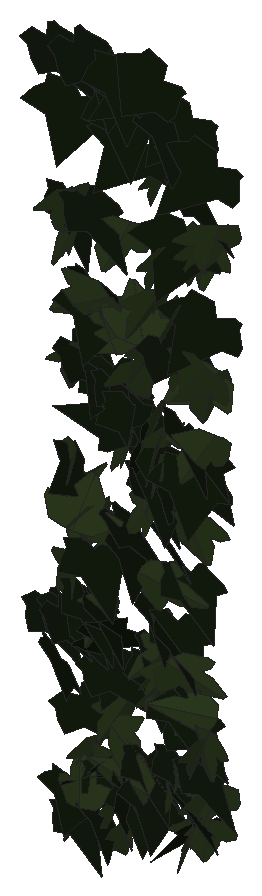
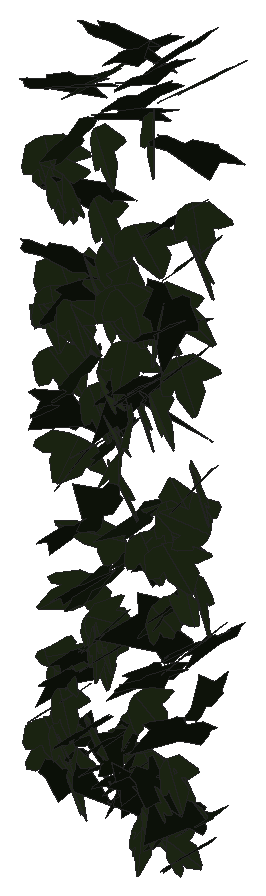
# SketchUp Ruby script. Lengths in inches.
U = 1.inch
M = Sketchup.active_model
def pt(a) = Geom::Point3d.new(a.map { |v| v * U })
def face(e, loops, mat)
  f = e.add_face(loops[0].map { |a| pt(a) })
  loops[1..].each { |l| e.add_face(l.map { |a| pt(a) }).erase! }
  f.material = f.back_material = mat if mat
  f
end
# faces: each face lists its corners as indices into pts; further lists are holes
def faces(e, pts, list, mat = nil) = list.each { |f| face(e, (f[0].is_a?(Array) ? f : [f]).map { |l| l.map { |i| pts[i] } }, mat) }
# xy, xz, yz: faces in a plane at the given z, y or x. An outline is a flat list of corners, or four numbers for a rectangle; further outlines are holes
def ring(l) = l.size == 4 ? [[l[0], l[1]], [l[2], l[1]], [l[2], l[3]], [l[0], l[3]]] : l.each_slice(2).to_a
def flat(e, list, mat, &to3) = list.each { |f| face(e, (f[0].is_a?(Array) ? f : [f]).map { |l| ring(l).map { |u, v| to3.(u, v) } }, mat) }
def xy(e, z, list, mat = nil) = flat(e, list, mat) { |x, y| [x, y, z] }
def xz(e, y, list, mat = nil) = flat(e, list, mat) { |x, z| [x, y, z] }
def yz(e, x, list, mat = nil) = flat(e, list, mat) { |y, z| [x, y, z] }
def lines(e, pts, list) = list.each { |a, b| e.add_line(pt(pts[a]), pt(pts[b])) }
# prism: a flat outline (further loops are holes) pulled along v
def prism(e, loops, v, mat = nil)
  f = face(e, loops, mat); d = Geom::Vector3d.new(v.map { |x| x * U })
  f.pushpull(f.normal.samedirection?(d) ? d.length : -d.length)
end
def box(e, o, s, mat = nil) = prism(e, [[o, [o[0] + s[0], o[1], o[2]], [o[0] + s[0], o[1] + s[1], o[2]], [o[0], o[1] + s[1], o[2]]]], [0, 0, s[2]], mat)
def at(x, y, z, deg = 0) = Geom::Transformation.translation(pt([x, y, z])) * Geom::Transformation.rotation(ORIGIN, Z_AXIS, deg.degrees)
def axes(o, x, y, z) = Geom::Transformation.new([*x, 0, *y, 0, *z, 0, *pt(o).to_a, 1])
def part(name) = M.definitions.add(name)
# library, detail: a bought-in or finely detailed component or shape, given as its bounding box
def library(name, o, s) = part(name).tap { |d| box(d.entities, o, s) }
def detail(e, o, s) = box(e.add_group.entities, o, s)
def put(e, d, t, mat = nil) = e.add_instance(d, t).tap { |i| i.material = mat if mat }
def group(e, t, mat = nil) = e.add_group.tap { |g| g.transformation = t; g.material = mat if mat }.entities
root = M.entities
M.materials.add("1026 AP 7946 SUNNY SIDE UP").color = [254, 231, 186]
M.materials.add("efeu1").color = [18, 25, 13]
M.materials.add("efeu2").color = [43, 57, 29]
c1 = part("ivyleaf_9")
p = [[1.54,2.16,1.25],[1.36,2.04,1.19],[-0.21,0.99,0.68],[-0.71,1.11,0.82],[-0.85,0.86,0.67],[-0.8,0.17,0.21],
  [-0.9,-0.01,0.1],[-0.67,-0.16,-0.02],[-0.08,-0.08,-0.05],[-0.03,-0.6,-0.4],[0.65,-0.88,-0.66],[0.83,-0.6,-0.49],
  [1.29,-0.42,-0.43],[1.8125,-0.07,-0.26],[1.21,0.44,0.15]]
faces(c1.entities,p,[[0,1,2,3,4,5,6,7,8,9,10,11,12,13,14]],"efeu1")
c2 = part("ivyleaf_10")
p = [[0,0.5,-0.03],[-0.0625,2.02,-0.43],[-0.19,2.01,-0.46],[-0.54,1.05,-0.29],[-0.52,0.625,-0.18],[-0.83,0.76,-0.28],
  [-1.16,0.64,-0.33],[-1.15,0.33,-0.24],[-0.77,-0.39,0.02],[-0.3,-0.51,0.16],[0.04,-0.48,0.23],[-0.02,2.01,-0.4375],
  [-0.06,2.01,-0.43],[0.04,-0.49,0.23],[0.67,-0.49,0.14],[1.38,0.36,-0.2],[1.375,0.51,-0.24],[0.81,0.65,-0.19],
  [0.62,0.59,-0.15],[0.6,1.09,-0.28],[0.5,1.23,-0.31]]
faces(c2.entities,p,[[0,1,2,3,4,5,6,7,8,9,10],[11,12,0,13,14,15,16,17,18,19,20]],"efeu2")
put(root,c1,axes([106.75,212.44,271.04],[0.09681,-0.2449,-0.11961],[-0.03354,0.11288,-0.25941],[0.42391,0.06486,0.00679]),"1026 AP 7946 SUNNY SIDE UP")
put(root,c1,axes([106.92,212.875,278.33],[-0.37251,-0.17456,-0.08374],[0.12341,0.02843,-0.30207],[0.27576,-0.24852,0.02207]),"1026 AP 7946 SUNNY SIDE UP")
put(root,c1,axes([106.76,212.92,276.76],[0.04968,-0.29311,0.04002],[0.0013,-0.04065,-0.30393],[0.46527,0.03141,-0.00342]),"1026 AP 7946 SUNNY SIDE UP")
put(root,c1,axes([106.68,212.56,279.28],[0.19725,-0.26448,-0.11631],[0.03527,0.13023,-0.29177],[0.44988,0.10575,0.07387]),"1026 AP 7946 SUNNY SIDE UP")
put(root,c1,axes([106.8,212.63,270.125],[0.01311,-0.18459,0.20212],[0.04458,-0.19565,-0.191],[0.42242,0.02638,0.01389]),"1026 AP 7946 SUNNY SIDE UP")
put(root,c2,axes([106.98,212.59,276.61],[0.27914,-0.2408,-0.00346],[-0.0098,-0.00212,-0.30814],[0.37851,0.17752,-0.00543]),"1026 AP 7946 SUNNY SIDE UP")
put(root,c2,axes([107.03,212.54,277.1],[-0.15174,-0.28317,-0.00569],[0.01853,0.00011,-0.30799],[0.44492,-0.09658,0.01089]),"1026 AP 7946 SUNNY SIDE UP")
put(root,c2,axes([107.09,212.42,271.66],[0.24519,-0.18142,-0.15122],[-0.08543,0.14222,-0.24141],[0.35581,0.15916,0.04624]),"1026 AP 7946 SUNNY SIDE UP")
put(root,c2,axes([107.04,212.52,273.27],[0.23828,-0.24035,-0.02918],[-0.00808,0.0286,-0.29233],[0.38021,0.15124,0.01207]),"1026 AP 7946 SUNNY SIDE UP")
put(root,c2,axes([106.96,212.6,272.6],[0.03462,-0.19119,0.23214],[0.01776,0.22743,0.19803],[-0.46564,-0.00554,0.02481]),"1026 AP 7946 SUNNY SIDE UP")
put(root,c2,axes([106.96,212.77,271.46],[0.03364,-0.25215,-0.12958],[0.0622,-0.12077,0.25858],[-0.43767,-0.03655,0.02679]),"1026 AP 7946 SUNNY SIDE UP")
put(root,c1,axes([106.93,212.47,270.97],[0.18903,-0.2168,-0.12971],[-0.06077,0.12057,-0.25367],[0.38852,0.12434,0.02343]),"1026 AP 7946 SUNNY SIDE UP")
put(root,c2,axes([107.2,212.875,272.26],[-0.26733,-0.18743,0.12168],[-0.05176,-0.12716,-0.25515],[0.34539,-0.16413,0.05594]),"1026 AP 7946 SUNNY SIDE UP")
put(root,c1,axes([106.9,212.61,270.99],[0.10787,-0.25178,-0.09699],[0.04478,0.102,-0.26303],[0.41952,0.05385,0.05302]),"1026 AP 7946 SUNNY SIDE UP")
put(root,c1,axes([107.03,212.63,268.27],[-0.10652,-0.21664,0.14167],[0.0268,-0.14694,-0.22865],[0.40364,-0.04742,0.05257]),"1026 AP 7946 SUNNY SIDE UP")
put(root,c2,axes([107.14,212.8,268.02],[0.02856,-0.18721,0.17963],[0.02622,-0.17463,-0.19479],[0.40256,0.02466,-0.00006]),"1026 AP 7946 SUNNY SIDE UP")
put(root,c2,axes([107.2,212.62,274.84],[-0.1653,-0.26983,0.04617],[-0.01409,-0.04623,-0.29848],[0.43027,-0.10518,0.00796]),"1026 AP 7946 SUNNY SIDE UP")
put(root,c1,axes([107.13,212.65,273.01],[-0.10645,-0.13164,0.24887],[-0.10943,-0.23329,-0.15195],[0.41958,-0.09424,0.02351]),"1026 AP 7946 SUNNY SIDE UP")
put(root,c1,axes([107,212.68,267.93],[0.07974,-0.25413,-0.0396],[0.00671,0.03854,-0.26647],[0.40375,0.04955,0.01225]),"1026 AP 7946 SUNNY SIDE UP")
put(root,c2,axes([107.49,212.56,275.73],[-0.28628,-0.0219,0.24485],[-0.35353,-0.08504,-0.1859],[0.12653,-0.28716,0.03455]),"1026 AP 7946 SUNNY SIDE UP")
put(root,c2,axes([107.27,212.72,269.04],[-0.03213,-0.26623,0.0073],[0.00325,-0.00878,-0.27511],[0.41883,-0.02036,0.00269]),"1026 AP 7946 SUNNY SIDE UP")
put(root,c1,axes([107.32,212.6875,275.82],[0.35562,0.01152,-0.20613],[-0.31415,-0.01219,-0.23336],[-0.02627,0.30176,0.00021]),"1026 AP 7946 SUNNY SIDE UP")
put(root,c1,axes([107.25,212.55,268.53],[0.2716,0.18112,0.07409],[0.02495,0.08137,-0.25353],[-0.30481,0.16805,0.04526]),"1026 AP 7946 SUNNY SIDE UP")
put(root,c2,axes([107.35,212.38,268.42],[0.41171,-0.05241,0.08667],[-0.11305,0.06435,0.27123],[-0.10787,-0.26748,0.04656]),"1026 AP 7946 SUNNY SIDE UP")
put(root,c1,axes([107.16,212.49,274.94],[0.20692,-0.22356,-0.15426],[-0.07258,0.14404,-0.26474],[0.4157,0.13643,0.03056]),"1026 AP 7946 SUNNY SIDE UP")
put(root,c1,axes([107.16,212.62,269.69],[0.04655,-0.16844,-0.21677],[0.0829,0.21027,-0.16529],[0.41443,-0.02315,0.05741]),"1026 AP 7946 SUNNY SIDE UP")
put(root,c1,axes([107.33,212.8125,275.47],[-0.18029,-0.2642,0.05893],[-0.00149,-0.06337,-0.29605],[0.42555,-0.11215,0.02393]),"1026 AP 7946 SUNNY SIDE UP")
put(root,c2,axes([107.43,212.82,274.32],[0.12232,-0.27329,0.0336],[0.00331,-0.03491,-0.29283],[0.43305,0.07746,-0.00725]),"1026 AP 7946 SUNNY SIDE UP")
put(root,c2,axes([107.47,212.52,272.61],[-0.06041,-0.28253,-0.0156],[0.01956,0.01196,-0.29346],[0.44433,-0.03894,0.0108]),"1026 AP 7946 SUNNY SIDE UP")
put(root,c1,axes([107.25,212.625,277.0625],[0.12157,-0.27918,-0.10473],[-0.00971,0.10188,-0.29712],[0.46624,0.07492,0.02112]),"1026 AP 7946 SUNNY SIDE UP")
put(root,c1,axes([107.6,212.74,268.91],[-0.16628,0.17993,-0.16113],[0.06189,-0.15669,-0.21265],[-0.3708,-0.10684,0.03676]),"1026 AP 7946 SUNNY SIDE UP")
put(root,c2,axes([107.36,212.27,272.57],[0.37983,0.14328,-0.10863],[0.11684,0.0818,0.28812],[0.255,-0.2509,0.0298]),"1026 AP 7946 SUNNY SIDE UP")
put(root,c1,axes([107.26,212.38,279.46],[0.20021,-0.2559,-0.16423],[-0.03168,0.1639,-0.28929],[0.47181,0.11959,0.05027]),"1026 AP 7946 SUNNY SIDE UP")
put(root,c2,axes([107.61,212.55,275.45],[-0.21205,0.20867,0.17767],[-0.17152,0.13302,-0.25464],[-0.38829,-0.17271,0.01545]),"1026 AP 7946 SUNNY SIDE UP")
put(root,c1,axes([107.35,212.49,271.37],[0.08721,-0.29426,-0.03799],[-0.018,0.03366,-0.30825],[0.46565,0.05641,-0.0048]),"1026 AP 7946 SUNNY SIDE UP")
put(root,c2,axes([107.59,212.74,268.62],[0.28842,-0.17099,-0.09848],[-0.07087,0.08925,-0.25566],[0.299,0.1861,0.03439]),"1026 AP 7946 SUNNY SIDE UP")
put(root,c2,axes([107.53,212.65,271.19],[-0.07298,-0.21554,0.18868],[0.07911,-0.19012,-0.21704],[0.43892,-0.00157,0.07049]),"1026 AP 7946 SUNNY SIDE UP")
put(root,c2,axes([107.78,212.58,268.89],[-0.31184,0.03947,0.17598],[-0.27306,-0.01122,-0.20536],[-0.03537,-0.26136,0.03383]),"1026 AP 7946 SUNNY SIDE UP")
put(root,c2,axes([107.72,212.6,278.22],[-0.21822,0.18572,0.2159],[-0.25315,0.13704,-0.23532],[-0.35874,-0.20967,0.03472]),"1026 AP 7946 SUNNY SIDE UP")
put(root,c1,axes([107.41,212.6875,268.06],[0.02727,-0.2283,0.13999],[0.02831,-0.13615,-0.23657],[0.41785,0.02412,0.00689]),"1026 AP 7946 SUNNY SIDE UP")
put(root,c2,axes([107.64,212.79,272.23],[-0.18987,-0.24116,0.085],[-0.00263,-0.09203,-0.27563],[0.40148,-0.11466,0.03839]),"1026 AP 7946 SUNNY SIDE UP")
put(root,c1,axes([107.53,212.77,274.64],[-0.14551,-0.24348,0.12868],[-0.01888,-0.12956,-0.26714],[0.43086,-0.08791,0.03175]),"1026 AP 7946 SUNNY SIDE UP")
put(root,c1,axes([107.48,212.51,272],[-0.04494,-0.2759,-0.08491],[0.00613,0.08088,-0.28525],[0.45203,-0.02853,-0.00457]),"1026 AP 7946 SUNNY SIDE UP")
put(root,c2,axes([107.71,212.82,276.69],[-0.29297,-0.20121,0.12071],[-0.03951,-0.13322,-0.27494],[0.3649,-0.17598,0.06715]),"1026 AP 7946 SUNNY SIDE UP")
put(root,c1,axes([107.6,212.91,270.33],[-0.17917,-0.23682,0.0624],[-0.01276,-0.0646,-0.27032],[0.38468,-0.11245,0.0201]),"1026 AP 7946 SUNNY SIDE UP")
put(root,c2,axes([107.625,212.74,268.24],[0.07756,-0.23671,0.11521],[0.04787,-0.10922,-0.24963],[0.40977,0.05756,0.00735]),"1026 AP 7946 SUNNY SIDE UP")
put(root,c1,axes([107.59,212.81,279.09],[-0.12225,-0.29427,0.05842],[-0.00316,-0.0598,-0.31362],[0.47172,-0.07666,0.01304]),"1026 AP 7946 SUNNY SIDE UP")
put(root,c1,axes([107.52,212.6,271.15],[0.0976,-0.2476,0.11251],[0.03804,-0.10797,-0.26359],[0.42472,0.06657,-0.00225]),"1026 AP 7946 SUNNY SIDE UP")
put(root,c1,axes([107.6,212.74,274.625],[-0.03427,-0.27213,-0.10131],[0.00324,0.09692,-0.28062],[0.45415,-0.02123,-0.00564]),"1026 AP 7946 SUNNY SIDE UP")
put(root,c1,axes([108.09,212.44,274.1],[-0.28269,0.16177,0.17135],[-0.25982,0.05685,-0.24197],[-0.25464,-0.23759,0.05666]),"1026 AP 7946 SUNNY SIDE UP")
put(root,c1,axes([107.56,212.61,270.38],[0.10212,-0.19481,-0.18732],[0.02517,0.18857,-0.20238],[0.41707,0.03632,0.05808]),"1026 AP 7946 SUNNY SIDE UP")
put(root,c2,axes([107.8,212.65,269.79],[-0.06915,-0.22701,0.15067],[0.00395,-0.14981,-0.23757],[0.4257,-0.03549,0.02668]),"1026 AP 7946 SUNNY SIDE UP")
put(root,c1,axes([107.63,212.72,268.78],[-0.06523,-0.21632,-0.16445],[0.03682,0.15675,-0.22593],[0.41997,-0.04734,-0.00573]),"1026 AP 7946 SUNNY SIDE UP")
put(root,c2,axes([107.77,212.68,267.97],[-0.03972,-0.24851,-0.09844],[0.0488,0.09116,-0.25595],[0.415,-0.0345,0.02068]),"1026 AP 7946 SUNNY SIDE UP")
put(root,c2,axes([107.95,212.67,275.4],[0.34033,0.06676,-0.19992],[-0.30198,-0.03509,-0.23285],[-0.11535,0.28883,0.01972]),"1026 AP 7946 SUNNY SIDE UP")
put(root,c1,axes([107.53,212.35,270.84],[0.26011,0.10348,0.21447],[0.29461,0.0907,-0.19986],[-0.21501,0.24946,-0.0144]),"1026 AP 7946 SUNNY SIDE UP")
put(root,c1,axes([107.69,212.6,268.33],[-0.22847,-0.00972,0.23143],[0.35096,0.02674,0.15003],[-0.04359,0.26625,-0.00504]),"1026 AP 7946 SUNNY SIDE UP")
put(root,c2,axes([107.83,212.63,268.16],[-0.13772,0.23085,0.07764],[-0.07386,0.06109,-0.25306],[-0.37399,-0.09708,0.02138]),"1026 AP 7946 SUNNY SIDE UP")
put(root,c2,axes([107.9,212.74,275.67],[-0.31001,-0.21954,0.04889],[-0.02807,-0.04928,-0.30362],[0.35249,-0.19701,0.01881]),"1026 AP 7946 SUNNY SIDE UP")
put(root,c1,axes([107.69,212.73,274.49],[0.09631,-0.27676,-0.06104],[0.02017,0.06168,-0.29048],[0.44406,0.05722,0.02643]),"1026 AP 7946 SUNNY SIDE UP")
put(root,c2,axes([107.9,212.82,273.94],[-0.13574,0.25031,-0.1234],[0.00189,-0.12657,-0.27091],[-0.4373,-0.07825,0.03713]),"1026 AP 7946 SUNNY SIDE UP")
put(root,c2,axes([108.03,212.84,275.69],[-0.25679,-0.22905,0.09314],[-0.02094,-0.10163,-0.28653],[0.38739,-0.15732,0.04625]),"1026 AP 7946 SUNNY SIDE UP")
put(root,c1,axes([107.73,212.64,272.55],[0.2663,-0.21234,-0.06948],[-0.00714,0.07993,-0.27548],[0.34968,0.16334,0.04729]),"1026 AP 7946 SUNNY SIDE UP")
put(root,c2,axes([108.28,212.38,268.86],[0.10402,0.05348,0.28183],[-0.43693,-0.00547,0.07037],[0.02829,-0.28111,0.05054]),"1026 AP 7946 SUNNY SIDE UP")
put(root,c1,axes([107.86,212.65,278.625],[-0.08869,-0.3052,-0.01569],[0.01486,0.01198,-0.31959],[0.48014,-0.05675,0.00699]),"1026 AP 7946 SUNNY SIDE UP")
put(root,c2,axes([107.96,212.41,269.52],[-0.022,0.24847,0.14552],[-0.02613,0.13907,-0.25544],[-0.44756,-0.02034,0.00776]),"1026 AP 7946 SUNNY SIDE UP")
put(root,c2,axes([108,212.72,274.84],[-0.17115,-0.2555,-0.09569],[0.08062,0.07737,-0.28517],[0.41901,-0.11925,0.01579]),"1026 AP 7946 SUNNY SIDE UP")
put(root,c1,axes([107.88,212.77,272.03],[-0.00759,-0.23191,0.16088],[0.00947,-0.15755,-0.23975],[0.44068,-0.00061,0.00792]),"1026 AP 7946 SUNNY SIDE UP")
put(root,c2,axes([108.08,212.38,273.96],[0.22534,-0.24614,-0.05372],[-0.03735,0.04488,-0.29315],[0.3934,0.14525,0.00293]),"1026 AP 7946 SUNNY SIDE UP")
put(root,c1,axes([107.95,212.53,279.22],[-0.09222,-0.30365,0.00616],[0.00664,-0.00866,-0.31859],[0.47757,-0.05852,0.00562]),"1026 AP 7946 SUNNY SIDE UP")
put(root,c1,axes([108.1,212.35,268.74],[0.12585,-0.06117,-0.27549],[-0.25564,0.21336,-0.09929],[0.34678,0.17948,0.02679]),"1026 AP 7946 SUNNY SIDE UP")
put(root,c2,axes([108.08,212.83,273.35],[-0.04153,0.26336,-0.11708],[-0.01341,-0.1163,-0.27269],[-0.45176,-0.02076,0.01886]),"1026 AP 7946 SUNNY SIDE UP")
put(root,c1,axes([108.2,212.6,278.22],[-0.34281,-0.1965,0.09413],[-0.03088,-0.11267,-0.29497],[0.34009,-0.2083,0.0681]),"1026 AP 7946 SUNNY SIDE UP")
put(root,c1,axes([107.96,212.72,268.73],[0.05757,-0.25442,0.08183],[0.02724,-0.0792,-0.2652],[0.4189,0.04011,0.006]),"1026 AP 7946 SUNNY SIDE UP")
put(root,c1,axes([108.04,212.6,274.28],[-0.05073,-0.28611,-0.05565],[0.00304,0.0525,-0.29628],[0.45735,-0.03208,-0.00421]),"1026 AP 7946 SUNNY SIDE UP")
put(root,c2,axes([108.27,212.59,272.92],[0.24703,-0.22255,-0.0814],[-0.10213,0.04896,-0.27927],[0.35633,0.16832,-0.02361]),"1026 AP 7946 SUNNY SIDE UP")
put(root,c2,axes([108.22,212.52,275.52],[0.42964,0.13671,0.02763],[-0.05645,0.0138,0.31348],[0.21142,-0.27413,0.02755]),"1026 AP 7946 SUNNY SIDE UP")
put(root,c1,axes([108.34,212.39,273.99],[0.0028,0.05486,-0.30194],[-0.28697,0.23238,0.04498],[0.3714,0.17914,0.03703]),"1026 AP 7946 SUNNY SIDE UP")
put(root,c2,axes([108.33,212.6,275.3125],[0.01982,-0.27548,0.10881],[-0.01058,-0.10752,-0.2845],[0.46468,0.0093,-0.01112]),"1026 AP 7946 SUNNY SIDE UP")
put(root,c1,axes([108.1875,212.58,268.61],[-0.08131,-0.25618,0.00065],[0.00607,-0.0029,-0.26922],[0.40279,-0.05167,0.00419]),"1026 AP 7946 SUNNY SIDE UP")
put(root,c1,axes([108.51,212.53,279.3],[-0.48129,-0.04339,0.0313],[-0.04127,-0.0322,-0.31735],[0.0726,-0.30593,0.02712]),"1026 AP 7946 SUNNY SIDE UP")
put(root,c2,axes([108.35,212.82,277.84],[0.03626,-0.30113,0.00252],[0.00199,-0.00408,-0.31116],[0.47354,0.02308,0.00112]),"1026 AP 7946 SUNNY SIDE UP")
put(root,c2,axes([108.4,212.53,276.05],[-0.06708,-0.26644,0.12767],[-0.02578,-0.12441,-0.27869],[0.46234,-0.0456,0.00298]),"1026 AP 7946 SUNNY SIDE UP")
put(root,c1,axes([108.09,212.74,269.01],[0.18729,-0.18383,0.16211],[0.11052,-0.14276,-0.22596],[0.36521,0.13747,-0.01476]),"1026 AP 7946 SUNNY SIDE UP")
put(root,c1,axes([108.26,212.77,270.43],[-0.01021,-0.26919,0.0476],[0.00428,-0.0478,-0.27765],[0.42986,-0.00591,0.00389]),"1026 AP 7946 SUNNY SIDE UP")
put(root,c1,axes([108.25,212.64,269.15],[0.02607,-0.26623,-0.02924],[0.01012,0.02731,-0.27452],[0.42063,0.01584,0.00841]),"1026 AP 7946 SUNNY SIDE UP")
put(root,c2,axes([108.37,212.7,274.33],[0.16127,-0.22997,0.14561],[0.06662,-0.13702,-0.25975],[0.42027,0.10997,-0.0147]),"1026 AP 7946 SUNNY SIDE UP")
put(root,c2,axes([108.47,212.71,270.81],[-0.04866,-0.11242,0.26008],[-0.01124,-0.25426,-0.11873],[0.43531,-0.01913,0.02601]),"1026 AP 7946 SUNNY SIDE UP")
put(root,c2,axes([108.33,212.72,273.86],[0.21084,-0.19621,0.17473],[0.1348,-0.148,-0.24546],[0.38611,0.15881,-0.00972]),"1026 AP 7946 SUNNY SIDE UP")
put(root,c1,axes([108.24,212.8,270.8],[0.17411,-0.24911,-0.05811],[-0.02754,0.05239,-0.28049],[0.40019,0.11199,0.00598]),"1026 AP 7946 SUNNY SIDE UP")
put(root,c2,axes([108.49,212.64,276.7],[0.0152,-0.29724,0.04817],[0.00582,-0.04835,-0.30665],[0.47351,0.01013,0.00222]),"1026 AP 7946 SUNNY SIDE UP")
put(root,c2,axes([108.51,212.73,274.02],[-0.06521,-0.27758,0.04023],[-0.00411,-0.04068,-0.28935],[0.4411,-0.04141,0.00325]),"1026 AP 7946 SUNNY SIDE UP")
put(root,c2,axes([108.49,212.58,270.62],[0.02821,-0.27374,-0.03139],[0.00204,0.02906,-0.28243],[0.43283,0.0177,0.00338]),"1026 AP 7946 SUNNY SIDE UP")
put(root,c2,axes([108.48,212.71,270.57],[0.02257,-0.2594,-0.09946],[0.03091,0.09592,-0.26599],[0.43332,0.00667,0.02415]),"1026 AP 7946 SUNNY SIDE UP")
put(root,c2,axes([108.4,212.55,273.61],[0.30634,-0.17505,0.13286],[0.12715,-0.10383,-0.26957],[0.31835,0.20991,-0.02017]),"1026 AP 7946 SUNNY SIDE UP")
put(root,c1,axes([108.3,212.54,273.41],[0.17391,-0.27551,-0.00378],[-0.013,-0.00105,-0.30574],[0.43303,0.11062,-0.00766]),"1026 AP 7946 SUNNY SIDE UP")
put(root,c1,axes([108.42,212.58,268.71],[-0.08698,-0.26579,0.07268],[0.00645,-0.07428,-0.27947],[0.43297,-0.05229,0.01876]),"1026 AP 7946 SUNNY SIDE UP")
put(root,c1,axes([108.375,212.72,271.35],[0.02689,-0.24562,0.13526],[0.00359,-0.13281,-0.25435],[0.43895,0.01613,-0.0062]),"1026 AP 7946 SUNNY SIDE UP")
put(root,c2,axes([108.57,212.55,270.36],[-0.04118,-0.27478,-0.02819],[-0.00099,0.02598,-0.28419],[0.43397,-0.02602,-0.00332]),"1026 AP 7946 SUNNY SIDE UP")
put(root,c2,axes([108.625,212.67,275.86],[0.1637,-0.2789,-0.01005],[-0.01338,0.00555,-0.30659],[0.43853,0.10428,-0.0056]),"1026 AP 7946 SUNNY SIDE UP")
put(root,c1,axes([108.35,212.79,272.43],[0.10406,-0.19469,0.20043],[0.11265,-0.1822,-0.21279],[0.41914,0.0973,0.00743]),"1026 AP 7946 SUNNY SIDE UP")
put(root,c2,axes([108.64,212.57,270.63],[-0.06171,-0.22979,0.15743],[0.01775,-0.15686,-0.2389],[0.43471,-0.02622,0.0321]),"1026 AP 7946 SUNNY SIDE UP")
put(root,c2,axes([108.68,212.5625,269.03],[0.24287,-0.24948,-0.07259],[-0.06482,0.05567,-0.3019],[0.40184,0.15977,-0.00482]),"1026 AP 7946 SUNNY SIDE UP")
put(root,c1,axes([108.67,212.96,278.61],[-0.3328,-0.20012,0.09083],[0.01382,-0.13181,-0.28359],[0.34429,-0.18814,0.09918]),"1026 AP 7946 SUNNY SIDE UP")
put(root,c1,axes([108.52,212.59,273.34],[-0.04521,-0.27852,0.0719],[0.01856,-0.07281,-0.28824],[0.45172,-0.02488,0.01904]),"1026 AP 7946 SUNNY SIDE UP")
put(root,c1,axes([108.55,212.71,278.59],[-0.05141,-0.28286,0.109],[0.03424,-0.10996,-0.29212],[0.47453,-0.02271,0.03288]),"1026 AP 7946 SUNNY SIDE UP")
put(root,c1,axes([108.625,212.66,273.27],[0.20449,-0.20364,-0.149],[-0.13374,0.11582,-0.2481],[0.36816,0.15518,-0.00737]),"1026 AP 7946 SUNNY SIDE UP")
put(root,c2,axes([108.43,212.53,271.93],[-0.09241,-0.02676,-0.28088],[0.41962,-0.06795,-0.05281],[-0.09632,-0.27035,0.03938]),"1026 AP 7946 SUNNY SIDE UP")
put(root,c2,axes([108.84,212.74,275.2],[-0.1164,-0.28415,0.02563],[-0.00173,-0.02708,-0.3026],[0.44873,-0.07381,0.00548]),"1026 AP 7946 SUNNY SIDE UP")
put(root,c1,axes([108.64,212.81,269.19],[0.01331,-0.27089,-0.00329],[-0.00078,0.00164,-0.2792],[0.42596,0.00847,-0.00041]),"1026 AP 7946 SUNNY SIDE UP")
put(root,c1,axes([108.82,212.72,277.01],[-0.38258,-0.17794,-0.05017],[0.0797,0.01129,-0.30975],[0.27849,-0.24768,0.01973]),"1026 AP 7946 SUNNY SIDE UP")
put(root,c1,axes([108.64,212.55,275.51],[0.08704,-0.16608,-0.25996],[0.00338,0.25582,-0.17211],[0.47376,0.02869,0.04899]),"1026 AP 7946 SUNNY SIDE UP")
put(root,c1,axes([108.67,212.73,271.26],[0.0225,-0.27497,-0.04171],[0.02234,0.03965,-0.28294],[0.4361,0.01216,0.01665]),"1026 AP 7946 SUNNY SIDE UP")
put(root,c1,axes([108.72,212.66,270.25],[-0.00506,-0.26204,-0.09566],[0.00473,0.09134,-0.26943],[0.43634,-0.00403,0.00181]),"1026 AP 7946 SUNNY SIDE UP")
put(root,c1,axes([108.67,212.62,271.13],[0.09549,-0.24462,0.12248],[0.05732,-0.11483,-0.26023],[0.42477,0.07049,0.00758]),"1026 AP 7946 SUNNY SIDE UP")
put(root,c2,axes([109.07,212.7,270.0625],[-0.00734,0.11704,0.25879],[-0.18103,-0.22865,0.10649],[0.39534,-0.10253,0.05357]),"1026 AP 7946 SUNNY SIDE UP")
put(root,c2,axes([108.89,212.7,268.26],[0.16009,-0.22964,0.07114],[0.0475,-0.06357,-0.25915],[0.37466,0.10618,0.00245]),"1026 AP 7946 SUNNY SIDE UP")
put(root,c2,axes([109.03,212.82,276.99],[-0.42539,0.13952,-0.02289],[-0.04941,-0.10776,-0.29307],[-0.21678,-0.24921,0.11172]),"1026 AP 7946 SUNNY SIDE UP")
put(root,c1,axes([108.75,212.75,277.74],[0.27036,-0.24598,-0.0563],[-0.02639,0.05314,-0.3084],[0.39486,0.17197,0.01794]),"1026 AP 7946 SUNNY SIDE UP")
put(root,c2,axes([109.13,212.75,275.05],[0.38352,0.00281,-0.17229],[-0.26281,-0.00785,-0.25129],[-0.01062,0.29564,-0.0033]),"1026 AP 7946 SUNNY SIDE UP")
put(root,c1,axes([109.12,212.66,268.49],[-0.15562,0.13654,-0.20598],[0.06364,-0.20444,-0.16503],[-0.37637,-0.09103,0.05726]),"1026 AP 7946 SUNNY SIDE UP")
put(root,c2,axes([109.03,212.72,269.46],[-0.03343,-0.26472,-0.00253],[0.0136,0.00026,-0.27345],[0.41603,-0.02128,0.00873]),"1026 AP 7946 SUNNY SIDE UP")
put(root,c1,axes([108.86,212.75,272.04],[0.00886,-0.27385,-0.07618],[0.00423,0.07245,-0.28172],[0.44537,0.00476,0.00419]),"1026 AP 7946 SUNNY SIDE UP")
put(root,c1,axes([108.84,212.72,269.91],[0.05814,-0.23051,-0.15206],[0.00906,0.14826,-0.23828],[0.42919,0.0281,0.02563]),"1026 AP 7946 SUNNY SIDE UP")
put(root,c1,axes([108.8125,212.67,274.2],[0.11584,-0.27652,0.11637],[0.03171,-0.1131,-0.29532],[0.46955,0.07586,-0.00876]),"1026 AP 7946 SUNNY SIDE UP")
put(root,c2,axes([109.1,212.72,277.02],[-0.02793,-0.29535,0.06152],[0.01052,-0.06187,-0.305],[0.47422,-0.01603,0.01039]),"1026 AP 7946 SUNNY SIDE UP")
put(root,c1,axes([108.84,212.69,273.79],[-0.11869,-0.14313,-0.24892],[0.2683,0.17431,-0.16081],[0.34935,-0.1825,0.03894]),"1026 AP 7946 SUNNY SIDE UP")
put(root,c1,axes([109.05,212.61,273.65],[-0.20496,-0.25491,-0.02945],[0.04607,0.01543,-0.29421],[0.40045,-0.13225,0.01878]),"1026 AP 7946 SUNNY SIDE UP")
put(root,c2,axes([109.08,212.47,273.01],[-0.4225,-0.05297,-0.0636],[0.10559,-0.02601,-0.27962],[0.07155,-0.2744,0.0371]),"1026 AP 7946 SUNNY SIDE UP")
put(root,c2,axes([109.15,212.65,268.89],[0.00148,-0.26777,0.04318],[0.00893,-0.04341,-0.27606],[0.42646,0.00184,0.00563]),"1026 AP 7946 SUNNY SIDE UP")
put(root,c1,axes([109.24,212.74,275.95],[-0.4301,-0.12074,-0.03032],[0.06009,-0.01574,-0.30659],[0.18567,-0.27459,0.02899]),"1026 AP 7946 SUNNY SIDE UP")
put(root,c2,axes([109.24,212.76,268.98],[-0.29095,-0.16764,0.08635],[-0.04519,-0.09232,-0.25326],[0.2919,-0.18139,0.04685]),"1026 AP 7946 SUNNY SIDE UP")
put(root,c2,axes([109.39,212.34,275.38],[-0.41095,0.04216,0.1576],[-0.24409,-0.00907,-0.27112],[-0.04995,-0.30258,0.02828]),"1026 AP 7946 SUNNY SIDE UP")
put(root,c2,axes([109.01,212.29,270.92],[-0.24212,-0.10733,-0.21645],[0.30532,0.08359,-0.19066],[0.20922,-0.24619,0.02775]),"1026 AP 7946 SUNNY SIDE UP")
put(root,c2,axes([109.31,212.53,274.23],[-0.23369,-0.20315,0.15179],[-0.04733,-0.15687,-0.25304],[0.39283,-0.13975,0.05981]),"1026 AP 7946 SUNNY SIDE UP")
put(root,c2,axes([109.27,212.59,268.53],[-0.30263,-0.17743,0.01889],[-0.00253,-0.02672,-0.26916],[0.28064,-0.19158,0.01794]),"1026 AP 7946 SUNNY SIDE UP")
put(root,c2,axes([109.19,212.58,269.84],[-0.35195,0.12958,-0.0636],[0.04136,-0.07673,-0.2615],[-0.22238,-0.21935,0.05202]),"1026 AP 7946 SUNNY SIDE UP")
put(root,c1,axes([108.98,212.5625,268.74],[0.08412,-0.20055,0.17891],[0.12686,-0.15768,-0.21272],[0.39863,0.0925,0.02994]),"1026 AP 7946 SUNNY SIDE UP")
put(root,c1,axes([109.36,212.59,278.3],[-0.3773,-0.17731,0.07941],[-0.05629,-0.08159,-0.30464],[0.2994,-0.23878,0.0428]),"1026 AP 7946 SUNNY SIDE UP")
put(root,c2,axes([109.28,212.43,269.83],[0.02327,-0.26513,0.01026],[0.00584,-0.01128,-0.27361],[0.41725,0.01494,0.00326]),"1026 AP 7946 SUNNY SIDE UP")
put(root,c2,axes([109.3,212.58,275.1],[-0.14088,-0.3068,-0.01659],[0.01893,0.01144,-0.32908],[0.48257,-0.09002,0.00806]),"1026 AP 7946 SUNNY SIDE UP")
put(root,c2,axes([109.35,212.64,277.3],[-0.22902,-0.2666,0.04058],[-0.00263,-0.0456,-0.31253],[0.4241,-0.14425,0.01998]),"1026 AP 7946 SUNNY SIDE UP")
put(root,c1,axes([109.12,212.5625,269.37],[0.12833,-0.24787,-0.07091],[0.00838,0.07237,-0.26699],[0.40383,0.07727,0.02807]),"1026 AP 7946 SUNNY SIDE UP")
put(root,c2,axes([109.32,212.49,268.85],[0.20218,-0.23792,0.04195],[0.01324,-0.04321,-0.27854],[0.37968,0.1282,-0.01262]),"1026 AP 7946 SUNNY SIDE UP")
